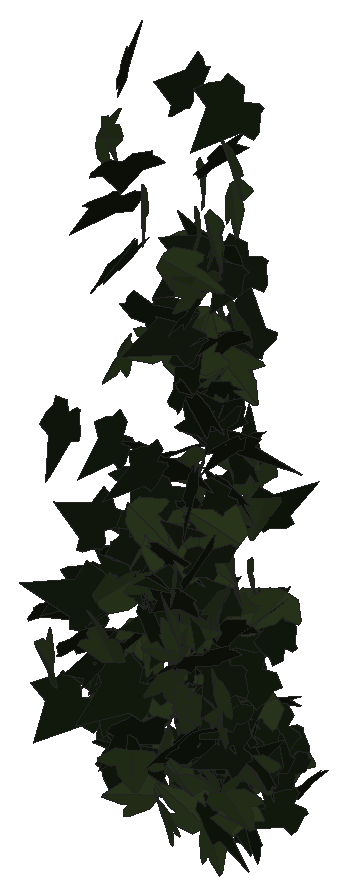
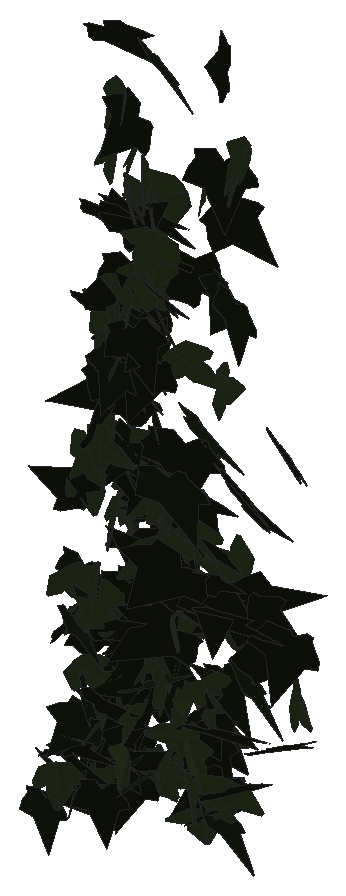
# SketchUp Ruby script. Lengths in millimetres.
U = 1.mm
M = Sketchup.active_model
def pt(a) = Geom::Point3d.new(a.map { |v| v * U })
def face(e, loops, mat)
  f = e.add_face(loops[0].map { |a| pt(a) })
  loops[1..].each { |l| e.add_face(l.map { |a| pt(a) }).erase! }
  f.material = f.back_material = mat if mat
  f
end
# faces: each face lists its corners as indices into pts; further lists are holes
def faces(e, pts, list, mat = nil) = list.each { |f| face(e, (f[0].is_a?(Array) ? f : [f]).map { |l| l.map { |i| pts[i] } }, mat) }
# xy, xz, yz: faces in a plane at the given z, y or x. An outline is a flat list of corners, or four numbers for a rectangle; further outlines are holes
def ring(l) = l.size == 4 ? [[l[0], l[1]], [l[2], l[1]], [l[2], l[3]], [l[0], l[3]]] : l.each_slice(2).to_a
def flat(e, list, mat, &to3) = list.each { |f| face(e, (f[0].is_a?(Array) ? f : [f]).map { |l| ring(l).map { |u, v| to3.(u, v) } }, mat) }
def xy(e, z, list, mat = nil) = flat(e, list, mat) { |x, y| [x, y, z] }
def xz(e, y, list, mat = nil) = flat(e, list, mat) { |x, z| [x, y, z] }
def yz(e, x, list, mat = nil) = flat(e, list, mat) { |y, z| [x, y, z] }
def lines(e, pts, list) = list.each { |a, b| e.add_line(pt(pts[a]), pt(pts[b])) }
# prism: a flat outline (further loops are holes) pulled along v
def prism(e, loops, v, mat = nil)
  f = face(e, loops, mat); d = Geom::Vector3d.new(v.map { |x| x * U })
  f.pushpull(f.normal.samedirection?(d) ? d.length : -d.length)
end
def box(e, o, s, mat = nil) = prism(e, [[o, [o[0] + s[0], o[1], o[2]], [o[0] + s[0], o[1] + s[1], o[2]], [o[0], o[1] + s[1], o[2]]]], [0, 0, s[2]], mat)
def at(x, y, z, deg = 0) = Geom::Transformation.translation(pt([x, y, z])) * Geom::Transformation.rotation(ORIGIN, Z_AXIS, deg.degrees)
def axes(o, x, y, z) = Geom::Transformation.new([*x, 0, *y, 0, *z, 0, *pt(o).to_a, 1])
def part(name) = M.definitions.add(name)
# library, detail: a bought-in or finely detailed component or shape, given as its bounding box
def library(name, o, s) = part(name).tap { |d| box(d.entities, o, s) }
def detail(e, o, s) = box(e.add_group.entities, o, s)
def put(e, d, t, mat = nil) = e.add_instance(d, t).tap { |i| i.material = mat if mat }
def group(e, t, mat = nil) = e.add_group.tap { |g| g.transformation = t; g.material = mat if mat }.entities
root = M.entities
M.materials.add("efeu1").color = [18, 25, 13]
M.materials.add("efeu2").color = [43, 57, 29]
c1 = part("ivyleaf_10")
p = [[0,12.8,-0.8],[-1.5,51.3,-10.9],[-4.9,51,-11.6],[-13.6,26.5,-7.3],[-13.2,15.9,-4.6],[-21.1,19.3,-7.2],
  [-29.5,16.3,-8.3],[-29.2,8.3,-6.2],[-19.7,-9.8,0.5],[-7.6,-13,4],[1,-12.2,5.8],[-0.4,51.1,-11.1],
  [-1.5,51.1,-10.9],[1,-12.4,5.9],[16.9,-12.4,3.5],[35.1,9.1,-5.1],[35,12.9,-6.1],[20.5,16.4,-4.9],
  [15.8,15,-3.8],[15.3,27.6,-7.1],[12.8,31.3,-7.8]]
faces(c1.entities,p,[[0,1,2,3,4,5,6,7,8,9,10],[11,12,0,13,14,15,16,17,18,19,20]],"efeu2")
c2 = part("ivyleaf_9")
p = [[39.1,54.8,31.7],[34.5,51.8,30.2],[-5.3,25.2,17.3],[-17.9,28.3,20.9],[-21.6,21.7,17],[-20.2,4.3,5.3],
  [-22.9,-0.3,2.5],[-17.1,-4,-0.6],[-2,-2.1,-1.2],[-0.7,-15.4,-10.1],[16.6,-22.3,-16.7],[21.1,-15.1,-12.5],
  [32.7,-10.7,-11],[46.1,-1.8,-6.6],[30.8,11.2,3.8]]
faces(c2.entities,p,[[0,1,2,3,4,5,6,7,8,9,10,11,12,13,14]],"efeu1")
put(root,c1,axes([489.6,867.5,1780.3],[-0.08629,0.03834,1.06216],[-1.14256,0.50111,-0.08045],[-0.61314,-0.93919,0.00043]))
put(root,c2,axes([488.7,875,1855.9],[0.44381,0.97962,0.1096],[0.07256,0.0948,-1.04474],[-1.20041,0.36791,-0.02263]))
put(root,c2,axes([498.2,902.7,1726.8],[-0.85353,-0.64794,0.3322],[0.00456,-0.46388,-0.89691],[0.88832,-0.62019,0.3238]))
put(root,c2,axes([498.5,978.3,1707.5],[-0.67587,-0.73439,0.18051],[-0.11573,-0.17104,-0.81552],[1.43463,-0.35977,0.01925]))
put(root,c2,axes([521.9,960.1,1665.2],[-0.54355,0.78411,0.05143],[-0.01127,0.05257,-0.83441],[-1.49548,-0.28539,-0.0124]))
put(root,c2,axes([503.6,876.3,2091.7],[-0.94055,0.02008,-0.65434],[0.78764,-0.14409,-0.76508],[-0.13226,-1.00087,0.09701]))
put(root,c1,axes([508.7,965.4,1701.1],[-1.41075,-0.3012,-0.23294],[0.4333,0.05803,-0.79952],[0.58087,-0.77482,0.03067]))
put(root,c2,axes([527.5,899.3,1888],[-0.02135,0.22308,-0.94051],[-0.1789,-0.93039,-0.21795],[-1.16561,0.13871,0.05068]))
put(root,c2,axes([529.6,962.6,1766.4],[-1.4171,-0.40023,0.0405],[0.117,-0.19741,-0.82066],[0.75661,-0.71908,0.20275]))
put(root,c2,axes([541.6,889.6,1799.8],[-0.79152,0.80027,0.11498],[-0.06841,0.10253,-1.03001],[-0.98398,-0.65087,-0.02088]))
put(root,c2,axes([513.5,968.5,1673.5],[-0.02001,-0.81612,-0.20319],[-0.03657,0.20338,-0.81591],[1.60023,-0.00556,-0.02119]))
put(root,c2,axes([536.8,911.5,2269.4],[-0.168,0.87962,0.41752],[-0.03646,0.41766,-0.88977],[-1.18733,-0.13729,-0.03175]))
put(root,c2,axes([542.2,921.2,2059.7],[-1.09858,0.24398,-0.18064],[0.21185,-0.04982,-0.93294],[-0.30379,-0.91706,0.00263]))
put(root,c2,axes([554.7,867.9,1878.5],[-0.46615,-0.03827,0.95633],[-1.16327,-0.07396,-0.38392],[0.10113,-1.02718,-0.00799]))
put(root,c1,axes([528.9,973.9,1666.1],[1.00727,0.64171,-0.07514],[-0.10859,-0.05033,-0.83172],[-1.22484,0.53218,0.01194]))
put(root,c2,axes([522.5,870,1813.3],[0.65826,0.76186,0.30871],[-0.21266,-0.25483,0.93356],[0.98007,-0.567,-0.00478]))
put(root,c2,axes([563.3,935.9,1887.2],[-1.49381,-0.15812,0.33707],[-0.60246,-0.13059,-0.79838],[0.373,-0.84417,0.06037]))
put(root,c1,axes([543.7,896.5,2443.6],[-0.72847,0.70119,0.36728],[-0.26247,0.29898,-0.92055],[-0.92934,-0.63407,-0.02791]))
put(root,c2,axes([549.1,919,1804.4],[-0.35363,0.78694,-0.427],[0.18474,-0.39926,-0.83862],[-1.07655,-0.32701,-0.00365]))
put(root,c1,axes([546,887.8,2445.3],[-0.00395,0.42152,0.9162],[-0.48068,0.84286,-0.38918],[-1.13261,-0.35918,0.16197]))
put(root,c2,axes([548.5,909.8,2276.1],[0.23243,0.67199,0.69095],[-0.0348,0.70794,-0.68065],[-1.17536,0.11193,0.15679]))
put(root,c1,axes([549.5,976.1,1699.2],[0.63814,-0.66129,-0.38228],[-0.08122,0.40061,-0.73044],[1.45145,0.31316,0.1272]))
put(root,c2,axes([559.3,896.7,2372.6],[-0.31743,0.66153,-0.69309],[-0.08324,-0.72916,-0.67034],[-1.16594,-0.12804,0.23656]))
put(root,c2,axes([549,928.9,1913.8],[0.78708,0.47543,-0.46119],[-0.45099,-0.27578,-0.8014],[-0.67054,0.74355,-0.00234]))
put(root,c1,axes([548.5,924.2,2169.1],[-0.19661,0.4278,-0.84597],[-0.20019,-0.85775,-0.40249],[-1.13909,0.0769,0.21676]))
put(root,c1,axes([551.4,968.8,1734.7],[0.14575,-0.84372,-0.04713],[0.01265,0.04792,-0.84712],[1.60822,0.07609,0.01093]))
put(root,c2,axes([571,852.7,1985],[-0.54948,0.48984,0.72061],[-0.6739,0.46684,-0.66258],[-0.82212,-0.71006,0.06149]))
put(root,c1,axes([550.8,949.9,1810.2],[0.67244,0.70703,-0.3529],[-0.41812,-0.28344,-0.78782],[-1.44463,0.41114,0.06375]))
put(root,c1,axes([568.9,865.6,1824.9],[-1.05529,0.13063,-0.387],[-0.46215,0.0824,0.8745],[0.18637,0.94403,-0.02278]))
put(root,c1,axes([562.8,943.6,1792.1],[1.02285,-0.30904,-0.2059],[-0.22708,0.09021,-0.89333],[0.39203,0.85859,0.01975]))
put(root,c2,axes([568.7,951.4,1761.2],[-0.48911,-0.50236,0.61577],[-0.31816,-0.56833,-0.63345],[0.91583,-0.46573,0.1088]))
put(root,c2,axes([571.9,888.7,2424.9],[0.36767,0.92296,-0.24577],[-0.10133,-0.23142,-0.97089],[-1.16083,0.31253,0.0069]))
put(root,c2,axes([571.2,953.7,1941.8],[-1.29156,-0.51522,-0.21541],[0.33149,0.12681,-0.85204],[1.0098,-0.70061,0.00419]))
put(root,c2,axes([558.6,909.8,1670.8],[-0.1105,-0.26221,-0.88706],[0.34469,0.84086,-0.2774],[1.07457,-0.29669,-0.00224]))
put(root,c2,axes([577.3,878.4,2534.6],[0.06233,-0.0036,0.99695],[0.28293,0.97092,-0.00838],[-1.18292,0.23203,0.05053]))
put(root,c2,axes([591.3,886.5,1785.1],[-1.24876,-0.15606,0.08121],[-0.07284,-0.14286,-1.02698],[0.2019,-1.0168,0.13182]))
put(root,c2,axes([592,893.4,1698.9],[0.40468,0.30094,-0.80444],[-0.85845,-0.39929,-0.43951],[-0.60087,0.77313,0.08614]))
put(root,c2,axes([588,900.4,1727.1],[-0.12277,0.56751,-0.79428],[0.05379,-0.79503,-0.57363],[-1.18974,-0.09451,0.05603]))
put(root,c1,axes([589.4,907.2,1638.4],[0.08477,0.22117,0.93813],[-0.20978,-0.92264,0.23025],[1.15704,-0.18349,-0.02699]))
put(root,c1,axes([585.5,950.9,1870.5],[0.20187,-0.86802,0.02616],[0.0651,-0.02215,-0.87392],[1.65148,0.10697,0.03125]))
put(root,c2,axes([597.6,950.7,2048.5],[0.06017,0.8889,-0.11605],[-0.17851,-0.11221,-0.885],[-1.69675,0.04333,0.08899]))
put(root,c1,axes([599.9,927,2192.3],[0.67802,0.13983,-0.73669],[-0.90934,0.00289,-0.56174],[-0.09989,0.9228,0.11339]))
put(root,c1,axes([579.3,854.6,1902.6],[-0.06156,-0.50908,0.85746],[0.18729,0.84436,0.51034],[-1.20208,0.15763,0.0356]))
put(root,c1,axes([589.5,962.9,1715.4],[-0.35407,0.8146,0.11247],[-0.06004,0.10185,-0.86467],[-1.00144,-0.29412,0.01207]))
put(root,c2,axes([577,960.9,1951.7],[1.55095,0.33541,0.00747],[0.01738,-0.00256,-0.88122],[-0.63827,0.81495,-0.00584]))
put(root,c1,axes([597.8,873.7,1701.3],[-0.99852,-0.50642,0.01917],[-0.01979,-0.01021,-0.96246],[0.61796,-0.81862,0.00015]))
put(root,c1,axes([574.4,946.2,1735.1],[0.21549,0.03919,0.87551],[0.99077,0.32841,-0.17854],[-0.40192,0.83058,0.02929]))
put(root,c1,axes([592.9,971.1,1802.7],[-0.60928,0.58873,-0.41896],[0.23886,-0.37999,-0.76734],[-0.84858,-0.52967,0.08482]))
put(root,c2,axes([607.6,922.5,2019],[-1.57947,-0.28092,-0.1811],[0.31306,0.07871,-0.8759],[0.55375,-0.84578,-0.02136]))
put(root,c2,axes([607.5,887.1,1897.8],[0.21263,-0.09987,1.01396],[-0.06093,1.02662,0.1097],[-1.24152,-0.06749,0.16827]))
put(root,c1,axes([610.5,914.1,1958.5],[0.58224,0.49761,-0.62637],[-0.62935,-0.36602,-0.68383],[-0.74593,0.69723,0.08804]))
put(root,c1,axes([602.3,887.1,2392.5],[-0.52528,0.71184,-0.53932],[0.10585,-0.56255,-0.81177],[-1.08439,-0.39972,0.18201]))
put(root,c2,axes([588.6,955.4,1867.5],[1.575,0.25066,0.12672],[0.21554,0.06301,-0.86426],[-0.48918,0.83482,0.02718]))
put(root,c2,axes([614.7,904.5,2065.4],[1.20624,0.33055,-0.55532],[-1.07442,-0.09539,-0.7011],[-0.59865,0.83724,0.13936]))
put(root,c1,axes([607.1,948,2040.8],[-0.54691,-0.74179,-0.41221],[0.37402,0.36521,-0.7942],[1.57121,-0.34514,0.04557]))
put(root,c2,axes([619.7,889,1952.7],[-0.968,0.44652,-0.24356],[0.25087,-0.13117,-0.91036],[-0.56755,-0.81955,0.01301]))
put(root,c2,axes([600.6,898.5,1953.6],[-1.13288,-0.24803,-0.60884],[1.20734,-0.00111,-0.61976],[0.32843,-0.85148,0.17816]))
put(root,c1,axes([630.7,921.6,1660.9],[0.36038,-0.03577,0.93929],[-1.13945,0.09987,0.29752],[-0.12933,-0.97956,-0.00396]))
put(root,c2,axes([617.6,931.4,1859.2],[-0.96408,-0.4265,-0.15279],[0.1651,0.07096,-0.89798],[0.52748,-0.80173,0.00181]))
put(root,c2,axes([627.1,874.2,2077.7],[-1.33998,0.42179,-0.39466],[0.54273,-0.28731,-0.81579],[-0.95605,-0.75427,0.09004]))
put(root,c2,axes([637.9,917.4,1872.3],[-0.99331,-0.05907,0.46775],[-0.56883,-0.03752,-0.81632],[0.08529,-0.93824,0.00319]))
put(root,c2,axes([606.7,887.1,1876.7],[0.80005,-0.62001,-0.26629],[-0.23947,0.18,-0.90247],[0.78763,0.68452,-0.00389]))
put(root,c1,axes([629.6,990.2,1706.8],[0.16164,0.33771,0.74564],[-0.61125,0.63078,-0.19666],[-0.78971,-0.41911,0.30484]))
put(root,c1,axes([618.7,979.2,1768.1],[-0.10124,0.82646,0.24025],[-0.00134,0.24126,-0.83032],[-1.05002,-0.07999,-0.02211]))
put(root,c1,axes([637.9,939.8,2031],[-0.53429,0.77431,0.37785],[-0.92871,0.18463,-0.7409],[-1.35142,-0.433,0.35977]))
put(root,c1,axes([620.9,906.5,1727.3],[-0.17839,0.19943,-0.87488],[0.0962,-0.88014,-0.21381],[-1.0905,-0.11027,0.12426]))
put(root,c2,axes([622.7,959.4,1786.9],[-0.72423,-0.65159,0.39941],[0.02498,-0.45169,-0.72437],[1.45434,-0.31672,0.21134]))
put(root,c1,axes([622.5,853.7,2020.1],[0.06169,0.77652,0.47703],[0.06554,0.47594,-0.7771],[-1.73322,0.04563,-0.01241]))
put(root,c1,axes([651.8,880.1,1849.8],[-0.42736,0.11795,0.91701],[-1.12638,0.00722,-0.35362],[-0.05963,-0.98161,0.10758]))
put(root,c2,axes([653.2,905.7,2536.7],[-0.6227,0.73188,0.45878],[-0.35771,0.35446,-0.89165],[-0.99125,-0.58767,0.03356]))
put(root,c2,axes([631.5,940.8,2177.6],[0.83716,0.58326,-0.16906],[-0.18743,-0.08006,-0.89979],[-0.71676,0.70217,0.03784]))
put(root,c2,axes([657.7,894.5,1840.1],[-0.37539,0.03101,-0.92375],[-1.12759,-0.01549,0.30734],[-0.00598,0.97352,0.03431]))
put(root,c2,axes([644.5,953.6,2219.9],[0.02865,0.84962,-0.38675],[-0.05374,-0.38543,-0.8494],[-1.1376,0.03961,0.03038]))
put(root,c1,axes([638.5,866,1942.9],[-0.7553,-0.77198,-0.28301],[0.21093,0.22412,-0.98955],[0.98068,-0.64276,-0.00513]))
put(root,c1,axes([636.5,901.2,1783.4],[-0.77571,0.74131,-0.05731],[0.04562,-0.04343,-0.97663],[-0.90595,-0.63692,-0.00011]))
put(root,c2,axes([617.2,875.1,2248.4],[-0.04149,-0.21356,0.95677],[1.06387,-0.44398,-0.0681],[0.54642,0.8482,0.20525]))
put(root,c1,axes([662.2,921.9,1666.7],[-0.34053,0.08871,-0.9003],[-1.05805,0.24188,0.29271],[0.31408,0.91101,0.00995]))
put(root,c1,axes([629.8,933.4,2327.5],[0.99728,0.29444,0.36822],[0.31859,0.33087,-0.84429],[-0.4789,0.83326,0.20514]))
put(root,c2,axes([659.4,936.3,1670.6],[-0.95555,-0.36423,-0.23745],[-0.26271,-0.10007,0.86379],[-0.46083,0.8123,-0.00006]))
put(root,c2,axes([643.1,921.4,2201.8],[0.38308,0.66158,0.60187],[0.09047,0.61643,-0.71627],[-1.0874,0.28435,0.15244]))
put(root,c1,axes([641.2,915.7,1992.8],[0.58606,0.74854,-0.25402],[-0.14513,-0.22541,-0.88918],[-0.95338,0.49445,-0.0208]))
put(root,c2,axes([650.7,890.9,1890.3],[0.00189,-0.14848,0.98461],[0.11895,0.97991,0.14762],[-1.20897,0.09618,0.01607]))
put(root,c1,axes([660.9,903.6,1636.2],[0.60159,0.20575,0.77948],[-0.89297,-0.26873,0.53397],[0.41226,-0.88234,0.01914]))
put(root,c2,axes([651.8,1000.5,1663.3],[0.14047,0.79053,-0.16015],[-0.0305,-0.1582,-0.79887],[-0.98357,0.1178,0.0019]))
put(root,c1,axes([646.8,933.1,2413.5],[0.66389,-0.72711,-0.33694],[0.00647,0.41054,-0.87737],[0.97767,0.49103,0.23461]))
put(root,c1,axes([640.1,915.4,1664.6],[-1.08725,0.16498,-0.40078],[0.47918,-0.08001,-0.90631],[-0.22355,-0.97388,0.00657]))
put(root,c2,axes([656.8,880.2,1835.5],[0.08971,1.04441,-0.04536],[-0.08428,-0.04052,-1.04491],[-1.2726,0.07631,0.066]))
put(root,c2,axes([659.5,855.6,1940.1],[0.53778,0.45301,-0.73059],[-0.83223,-0.31529,-0.60708],[-0.6382,0.79288,0.17602]))
put(root,c1,axes([651.1,857.9,1664.2],[-0.95261,0.60175,0.16888],[-0.15612,0.1106,-0.98575],[-0.74634,-0.79119,-0.00935]))
put(root,c2,axes([633.5,975.2,1663.5],[0.24388,-0.82287,0.0192],[-0.0241,-0.0214,-0.83264],[1.56632,0.1278,-0.0158]))
put(root,c2,axes([668.2,989.9,1761.9],[-0.24188,0.34186,0.72642],[-0.80968,0.35125,-0.34644],[-0.55115,-0.66605,0.19014]))
put(root,c1,axes([636.9,870.6,1984.2],[0.36201,0.63575,0.71383],[0.39121,0.63792,-0.70144],[-1.09862,0.43665,-0.01456]))
put(root,c1,axes([647.7,926.1,1795.3],[-0.35609,0.84168,-0.10173],[0.06077,-0.09038,-0.89068],[-1.03254,-0.29559,-0.01734]))
put(root,c1,axes([651.3,866,1913.3],[-0.61003,0.94653,0.04891],[-0.02183,0.04586,-1.07047],[-1.1561,-0.50032,-0.00559]))
put(root,c2,axes([660.7,981.4,1855.9],[-0.79025,-0.49461,0.22946],[-0.2103,-0.15228,-0.81484],[0.63108,-0.6701,0.0158]))
put(root,c1,axes([664,901.6,2364.2],[0.28972,-0.57909,-0.77378],[-0.36982,0.71196,-0.62585],[1.11961,0.38502,-0.0065]))
put(root,c2,axes([658.7,962.9,2178],[0.23886,0.81669,0.3692],[0.07566,0.36466,-0.83952],[-1.09082,0.20413,0.02262]))
put(root,c2,axes([677,887.5,2230.2],[-0.2904,0.54178,0.76344],[-0.7398,0.5109,-0.55163],[-0.8701,-0.6152,0.21422]))
put(root,c1,axes([657.2,869,1828],[-0.40341,-0.91612,-0.35897],[0.14038,0.34009,-0.97394],[1.19216,-0.35005,-0.00678]))
put(root,c2,axes([675.7,873.6,2263.1],[-1.24851,0.02852,0.26005],[-0.31759,-0.00706,-1.02367],[-0.0316,-1.05587,0.01387]))
put(root,c2,axes([667.6,859,1747.3],[-0.09244,1.08266,0.05384],[-0.01875,0.0529,-1.08525],[-1.32235,-0.07644,0.01162]))
put(root,c1,axes([658.4,948.5,2248.9],[-0.72038,0.7259,0.0234],[-0.06493,-0.01317,-0.93442],[-0.88368,-0.59079,0.04958]))
put(root,c2,axes([676.3,923.1,2193.3],[-0.75103,0.73662,0.11423],[-0.08626,0.08978,-0.95998],[-0.90532,-0.61964,-0.00329]))
put(root,c2,axes([643.6,857.5,1980.8],[1.19423,-0.06898,0.12471],[0.15196,-0.00655,-0.9813],[0.0845,0.98676,0.0022]))
put(root,c2,axes([676.8,865.6,2185.5],[-0.04664,0.42167,0.97575],[-0.33114,0.94014,-0.41691],[-1.25382,-0.26398,0.07382]))
put(root,c2,axes([667.2,910.6,1745.5],[0.75469,0.02599,-0.70031],[-0.85496,0.02539,-0.61808],[0.00225,0.93405,0.03629]))
put(root,c1,axes([651,885.5,1945.5],[0.11522,-0.17868,0.97324],[0.72609,-0.7708,-0.19927],[0.96443,0.60165,0.03375]))
put(root,c1,axes([668,958.4,2167.2],[-0.5222,0.64043,0.51265],[-0.33777,0.43153,-0.77025],[-0.94209,-0.50971,-0.00799]))
put(root,c1,axes([659.5,899.2,1866.6],[0.35958,-0.66877,0.64401],[0.31525,-0.5899,-0.73083],[1.08794,0.39197,-0.00108]))
put(root,c1,axes([667.4,924.4,2155.7],[0.80716,-0.81769,-0.1481],[0.03479,0.17541,-0.91614],[1.58117,0.41356,0.09576]))
put(root,c2,axes([652.8,950.5,1671.5],[0.34937,-0.78905,0.23918],[0.12181,-0.21814,-0.8392],[0.99849,0.3027,0.01869]))
put(root,c2,axes([679.8,935,1801.4],[-0.45707,-0.80415,-0.06824],[0.00993,-0.079,0.88622],[-0.98454,0.37253,0.04062]))
put(root,c2,axes([656.7,941.6,1710],[-0.0004,-0.53595,-0.70786],[0.15688,0.70037,-0.53033],[1.07178,-0.10271,0.07736]))
put(root,c2,axes([650.1,945.9,1783.6],[0.93022,-0.40376,0.16957],[0.18491,-0.07612,-0.86277],[0.50125,0.77738,0.00359]))
put(root,c1,axes([665.4,987,1736],[-0.13945,0.81485,-0.0705],[0.00201,-0.07096,-0.82279],[-0.99783,-0.11402,0.00819]))
put(root,c2,axes([644.9,915.2,2000.3],[0.75449,0.19992,-0.65752],[0.68112,0.36966,0.6375],[0.48892,-0.82349,0.12654]))
put(root,c2,axes([684.1,921.3,2316.9],[0.36213,-0.2504,0.90511],[-0.90251,0.52241,0.38713],[-0.70578,-0.7965,-0.03063]))
put(root,c2,axes([667.7,926.7,1648.2],[0.90447,0.41652,-0.33452],[-0.34314,-0.18216,-0.85014],[-0.55411,0.79269,-0.01959]))
put(root,c1,axes([680,873.5,1802.4],[-1.23468,-0.03048,0.33589],[-0.40925,-0.01922,-1.01245],[0.04268,-1.06614,0.00865]))
put(root,c1,axes([691.1,935.1,2175.3],[0.02834,0.09075,0.95466],[-1.16633,0.07709,0.01593],[-0.09176,-0.95183,0.09231]))
put(root,c2,axes([653.6,898.6,1893.6],[-0.21321,-0.09602,0.92837],[1.13865,-0.01938,0.17369],[0.00169,0.94447,0.09795]))
put(root,c2,axes([663,927.1,1767.3],[-0.31435,-0.78685,-0.38038],[0.16188,0.35675,-0.82785],[1.05388,-0.2895,0.0137]))
put(root,c1,axes([669,892.1,2250.3],[-0.59225,-0.7056,-0.43436],[0.29291,0.36204,-0.85644],[0.9675,-0.54153,-0.00661]))
put(root,c1,axes([667.9,897.7,1822.4],[0.59777,0.78036,-0.26153],[0.1798,0.21626,0.92138],[0.98785,-0.51157,-0.00944]))
put(root,c1,axes([660.4,891.5,1911.6],[-0.42053,-0.41366,-0.79733],[0.70273,0.55352,-0.53618],[0.84089,-0.66945,0.04934]))
put(root,c1,axes([662.2,915.2,1756.5],[0.42923,0.74282,0.48682],[0.25557,0.43945,-0.82192],[-1.05295,0.40947,-0.00104]))
put(root,c1,axes([662.8,905.9,1780.7],[1.00732,-0.34136,0.33469],[0.36924,-0.14381,-0.89331],[0.45148,0.87924,-0.01616]))
put(root,c2,axes([681.4,970.1,1845.5],[-0.88301,-0.44948,0.19428],[-0.20128,-0.10259,-0.85199],[0.56247,-0.74234,0.00011]))
put(root,c1,axes([666.4,892.1,2261.8],[0.89627,0.60201,0.14105],[0.14388,0.0786,-0.9497],[-0.7405,0.74393,-0.0138]))
put(root,c2,axes([692.2,903.7,2337.3],[-1.79023,-0.1192,-0.01452],[0.04911,-0.08869,-0.94377],[0.2232,-0.93656,0.09122]))
put(root,c2,axes([685.2,874.7,2301.1],[-0.82066,0.60958,-0.30603],[0.29562,-0.18822,-0.90752],[-0.77787,-0.71465,-0.02202]))
put(root,c2,axes([696.4,887.5,1956],[-1.01522,-0.05968,0.62281],[-0.7246,-0.25048,-0.81757],[0.23998,-1.00877,0.16616]))
put(root,c2,axes([680,919.4,1873.9],[0.5318,0.73963,-0.28028],[-0.25051,-0.20323,-0.85566],[-0.93188,0.47672,0.07007]))
put(root,c2,axes([663.5,877.6,1734.6],[0.71131,0.47403,0.66189],[0.63154,0.4125,-0.75141],[-0.7666,0.77966,-0.00487]))
put(root,c1,axes([699.8,952,2061.4],[-0.18441,0.0275,0.90868],[-1.09885,-0.12943,-0.14591],[0.15039,-0.91203,0.0481]))
put(root,c1,axes([684.2,970.9,1911.7],[-0.60908,0.61751,0.39235],[-0.36262,0.26284,-0.79188],[-0.81559,-0.57801,0.05907]))
put(root,c2,axes([677.3,909.3,2455],[0.35026,0.71555,0.64589],[0.30915,0.5942,-0.77092],[-1.13465,0.38278,-0.01066]))
put(root,c2,axes([684.7,907,2130.1],[0.61398,0.16234,0.84395],[-0.98537,-0.24489,0.52874],[0.35832,-0.95161,0.00791]))
put(root,c1,axes([664.7,982.2,1869.4],[0.44939,0.27576,0.71285],[0.62169,0.50119,-0.45719],[-0.695,0.62662,0.05197]))
put(root,c1,axes([692.5,936.8,2252.8],[-0.87088,0.38656,0.51369],[-0.60153,0.16341,-0.80812],[-0.50332,-0.86414,0.07698]))
put(root,c2,axes([695.2,894.5,2003.1],[-0.84185,0.61843,-0.06955],[0.05739,-0.05171,-0.92658],[-0.75706,-0.6916,0.00709]))
put(root,c2,axes([674.3,882.5,2071.3],[-0.52006,0.09124,-0.85782],[0.96761,-0.33489,-0.42975],[-0.41395,-0.89744,0.07316]))
put(root,c2,axes([696.2,1013.8,1712.5],[-0.8982,-0.13506,0.33056],[-0.38298,-0.11623,-0.74666],[0.20764,-0.79862,0.05276]))
put(root,c2,axes([677.3,998.5,1744.4],[0.74506,0.50027,0.21872],[0.02807,0.30429,-0.76022],[-0.66552,0.57289,0.21279]))
put(root,c1,axes([685.8,930.3,2165.7],[0.2684,-0.68346,-0.59855],[0.02854,0.60739,-0.69002],[1.72883,0.09608,0.10432]))
put(root,c1,axes([688.5,879.2,2310.2],[-0.53184,-0.46998,-0.78449],[-0.40675,-0.72757,0.62115],[-1.0389,0.52546,0.15841]))
put(root,c1,axes([682.2,915,2360.9],[0.54013,-0.8795,0.1597],[0.10989,-0.13341,-0.98444],[1.08499,0.45135,0.02021]))
put(root,c2,axes([696.6,997.9,1866.2],[-0.63484,0.67298,0.02417],[-0.01511,0.02097,-0.85068],[-0.82142,-0.5205,-0.00303]))
put(root,c2,axes([679.9,903.5,2174.8],[0.88149,0.58524,-0.09618],[-0.09188,-0.05983,-0.92982],[-0.71772,0.72645,0.00091]))
put(root,c1,axes([674.6,955.4,1865.9],[-0.00914,-0.14571,0.87284],[0.30824,0.83619,0.14176],[-1.03466,0.2504,0.03453]))
put(root,c2,axes([703.6,901.1,2135.4],[-0.6732,0.63144,0.38447],[-0.34769,0.26099,-0.83767],[-0.83222,-0.61983,0.03896]))
put(root,c1,axes([663.8,878.6,1886.7],[-0.4504,-0.06357,0.93024],[1.13684,0.00994,0.37049],[-0.0399,1.00077,0.0554]))
put(root,c1,axes([678.6,885.4,2222.7],[1.21407,-0.27811,-0.08585],[0.11427,0.01645,1.03246],[-0.33621,-0.9987,0.04092]))
put(root,c2,axes([691,877.3,1857.4],[0.35015,0.87565,-0.16655],[-0.09313,-0.15018,-0.92114],[-1.08345,0.2959,0.02535]))
put(root,c1,axes([680.7,942.2,1653.6],[0.07385,-0.10299,0.88676],[0.08925,0.88638,0.09795],[-1.08545,0.06587,0.06838]))
put(root,c1,axes([666.3,859.9,2343.8],[-0.5105,0.00511,-0.92472],[1.12806,-0.01195,-0.41848],[-0.01585,-1.01492,0.00027]))
put(root,c2,axes([706.3,986.7,1673.1],[-0.29799,0.32299,0.75742],[-0.65576,0.53596,-0.40188],[-0.76101,-0.5883,0.04972]))
put(root,c2,axes([700.4,906.9,2046.1],[-1.08585,0.34188,-0.12334],[0.13647,-0.05275,-0.9534],[-0.42188,-0.897,0.00906]))
put(root,c2,axes([686.1,902.1,1927.7],[-0.65877,-0.74652,-0.13099],[0.10007,0.10233,-0.92131],[0.91924,-0.54613,0.00642]))
put(root,c2,axes([679.4,921,2052.4],[1.09263,-0.04438,-0.25493],[-0.31065,0.01244,-0.8967],[0.05623,0.93109,-0.00017]))
put(root,c2,axes([676,926.6,1733.7],[-0.38013,-0.00758,0.87739],[1.06986,0.02833,0.31167],[-0.03566,0.93064,-0.00234]))
put(root,c2,axes([692.5,981.7,1677.4],[0.53162,-0.12541,-0.70487],[-0.7711,0.3202,-0.4477],[0.41026,0.76433,0.0719]))
put(root,c1,axes([694.9,926.6,2183.7],[-0.46827,-0.85515,0.18299],[0.01361,-0.20461,-0.93279],[1.06682,-0.37275,0.09223]))
put(root,c1,axes([678.3,914.5,2354.7],[0.77749,-0.45419,0.59866],[0.6365,-0.2975,-0.7811],[0.6598,0.8222,0.04808]))
put(root,c2,axes([715.4,865.4,1990.9],[-0.30797,0.27697,0.87213],[-0.93931,0.42462,-0.3577],[-0.60329,-0.80252,0.11173]))
put(root,c1,axes([696.3,966.7,2055.3],[0.08996,0.86154,-0.25574],[-0.37699,-0.21665,-0.81894],[-1.02956,0.15461,0.27753]))
put(root,c2,axes([699.5,904.6,1764],[-0.82488,-0.43593,0.43437],[0.43988,0.24235,0.80445],[-0.60843,0.76623,-0.00731]))
put(root,c2,axes([682.5,935.6,1684.9],[0.17936,0.08202,0.89432],[0.84243,0.5691,-0.16571],[-0.70054,0.70537,0.0297]))
put(root,c2,axes([683.9,940.5,1657.9],[-0.58246,-0.28754,-0.72092],[0.7597,0.36331,-0.55729],[0.56521,-0.78464,0.00614]))
put(root,c2,axes([699.8,937.2,2221],[-1.09163,0.0678,0.30911],[0.3764,-0.0194,0.89734],[0.08591,0.94647,-0.00375]))
put(root,c2,axes([691.5,983.7,1766.7],[-0.52679,0.21164,-0.70348],[0.76688,-0.31587,-0.48086],[-0.46384,-0.7626,0.00393]))
put(root,c2,axes([696.6,855.4,2191.5],[0.95085,0.02062,-0.64117],[-0.78136,-0.0325,-0.77957],[-0.04461,1.00871,-0.01201]))
put(root,c2,axes([703.8,885.8,2252],[0.19447,0.87779,-0.31583],[-0.12241,-0.30242,-0.89115],[-1.13152,0.18358,0.04213]))
put(root,c1,axes([703.7,955.8,2047.3],[-0.54891,-0.59437,-0.53274],[-0.3945,-0.42339,0.74546],[-0.8903,0.55407,-0.00186]))
put(root,c1,axes([699.5,899.2,1772.7],[-0.44721,0.77591,0.31223],[-0.15894,0.28377,-0.85813],[-1.00792,-0.38902,-0.00321]))
put(root,c1,axes([714.6,874.3,1914.6],[-0.07947,0.27241,0.89044],[-0.94227,0.48281,-0.2042],[-0.63459,-0.75101,0.1917]))
put(root,c2,axes([698,913.1,1830.3],[-0.42658,-0.78655,0.29494],[-0.13963,-0.27189,-0.86075],[1.01529,-0.36786,0.00555]))
put(root,c2,axes([695.4,1014.3,1708.7],[-0.48437,-0.71602,0.01437],[0.16665,-0.09184,-0.80214],[0.85768,-0.38652,0.16397]))
put(root,c1,axes([703.5,1015.8,1676.2],[-0.75024,-0.52078,0.05718],[-0.02068,-0.06834,-0.80479],[0.63884,-0.61381,0.04109]))
put(root,c1,axes([707.7,882.9,1821.8],[-0.99712,0.56001,0.17259],[-0.35968,-0.13697,-0.95169],[-0.61785,-0.82403,0.27548]))
put(root,c2,axes([705.5,940.3,2065.6],[-0.32139,-0.52387,0.74316],[0.3994,0.66718,0.58636],[-1.03488,0.42018,-0.00449]))
put(root,c2,axes([693.3,860.1,1965.9],[0.28432,0.76695,0.52291],[-0.23365,-0.48781,0.80083],[1.1081,-0.29964,0.03469]))
put(root,c2,axes([713,851,1789.8],[0.06235,0.96688,0.22476],[-0.16121,0.22968,-0.95801],[-1.20027,0.01938,0.14035]))
put(root,c1,axes([703.5,916,2418.3],[-0.18975,0.96808,0.05591],[-0.20145,0.02935,-0.96766],[-1.16575,-0.16265,0.15812]))
put(root,c1,axes([716.9,955.9,1775.1],[0.49817,0.21576,-0.7096],[-0.81568,-0.24356,-0.45879],[-0.39168,0.78164,0.05292]))
put(root,c2,axes([715.1,944.9,1819.4],[-0.03512,-0.25717,-0.90601],[-0.13838,-0.89889,0.25875],[-1.14063,0.11697,-0.0035]))
put(root,c2,axes([722.7,996.1,1670.6],[-0.40131,0.58478,0.46485],[-0.46792,0.30366,-0.65341],[-0.78208,-0.48175,0.15241]))
put(root,c2,axes([712.9,1023.3,1641.2],[-0.01776,0.79464,0.0476],[0.00553,0.04769,-0.79475],[-0.97118,-0.01426,-0.0054]))
put(root,c1,axes([686.3,865.8,1988.2],[0.52825,0.25024,0.81071],[0.83906,0.4295,-0.49989],[-0.60617,0.81257,0.01456]))
put(root,c1,axes([702.4,908.4,2474.3],[-0.82721,0.68925,-0.21859],[0.16352,-0.17466,-0.9665],[-0.86687,-0.69067,0.02628]))
put(root,c1,axes([680.9,915.3,2210.4],[1.39248,0.15383,0.57334],[1.03696,0.1872,-0.74551],[-0.44846,0.91049,0.05641]))
put(root,c2,axes([676.7,910.4,2112.6],[1.54878,0.08466,0.41578],[0.78823,0.03703,-0.81815],[-0.17557,0.91309,-0.00537]))
put(root,c1,axes([712.9,954.1,2019],[-0.47271,-0.83117,0.14025],[-0.07694,-0.12534,-0.91704],[1.02548,-0.39254,-0.00415]))
put(root,c2,axes([713.3,925,2338.3],[-1.07824,-0.3506,-0.16234],[0.20327,0.01982,-0.94985],[0.42528,-0.89837,0.0424]))
put(root,c1,axes([712.4,902.5,1954],[-0.66406,0.64498,0.34261],[-0.28894,0.24832,-0.84374],[-0.84285,-0.59329,0.01931]))
put(root,c2,axes([721.1,922.4,1638.6],[0.3052,-0.00382,-0.87619],[-1.06858,0.02336,-0.25018],[0.02868,0.91091,0.00274]))
put(root,c2,axes([721.5,993.1,1633.7],[-0.93406,-0.13707,0.21901],[-0.2609,-0.04815,-0.77774],[0.17688,-0.79488,0.00934]))
put(root,c1,axes([707.8,912.8,1665.3],[0.70099,0.62679,-0.25093],[-0.21098,-0.18187,-0.85029],[-0.79621,0.60003,0.00439]))
put(root,c2,axes([717.8,982.8,1834.1],[-0.35791,-0.7251,0.4018],[0.18126,0.37333,0.7822],[-0.99499,0.32884,-0.00204]))
put(root,c1,axes([707.4,871.4,2399.3],[-0.47677,0.89199,-0.03382],[0.02292,-0.02869,-0.97383],[-1.08877,-0.3912,-0.00569]))
put(root,c1,axes([727.6,876.7,2019.5],[0.45969,0.34332,0.82398],[-0.89218,-0.39416,0.49864],[0.6245,-0.81582,0.10584]))
put(root,c2,axes([722,903.2,2125.4],[-0.27615,0.71247,-0.5332],[-0.04094,-0.55662,-0.72952],[-1.0849,-0.16035,0.16324]))
put(root,c2,axes([699,877.2,1669.6],[0.87492,-0.65764,-0.35551],[-0.28591,0.27004,-0.97229],[0.86608,0.75351,0.03816]))
put(root,c1,axes([710.7,867.9,1649.6],[-0.03967,1.02405,0.21124],[-0.16229,0.20557,-1.01705],[-1.26527,-0.05848,0.12383]))
put(root,c1,axes([709,935.8,1704.7],[-0.89278,-0.35797,-0.32384],[0.3409,0.16543,-0.8143],[0.48021,-0.78295,-0.02399]))
put(root,c2,axes([729.3,896.3,1749],[-1.00027,0.324,0.15755],[-0.18513,0.04463,-0.88148],[-0.39865,-0.8337,0.01405]))
put(root,c2,axes([724.6,901,2546.8],[-1.12358,-0.39666,0.0533],[-0.06047,-0.01966,-1.00276],[0.48452,-0.9223,-0.00155]))
put(root,c1,axes([721.6,972,1896.3],[0.63389,0.48892,-0.49857],[-0.56053,-0.22863,-0.703],[-0.64154,0.68284,0.12161]))
put(root,c2,axes([726,940.6,1891.9],[0.0192,0.82906,0.25265],[-0.12018,0.25277,-0.8233],[-1.05052,-0.01376,0.0988]))
put(root,c1,axes([717.1,893,1683.9],[-0.92309,-0.34763,-0.33872],[0.37147,0.14858,-0.83263],[0.46113,-0.81556,-0.00731]))
put(root,c1,axes([723.2,871.5,1947],[0.15129,-0.92503,0.0834],[0.00196,-0.08393,-0.93326],[1.13311,0.12365,-0.00952]))
put(root,c2,axes([718.6,941,1708.4],[0.65901,-0.75662,-0.18939],[0.13667,-0.15273,0.92966],[-0.94169,-0.55166,0.00238]))
put(root,c2,axes([708.7,961,2001.1],[0.01356,-0.03866,0.90995],[1.00712,0.38487,0.00627],[-0.46941,0.82462,0.03973]))
